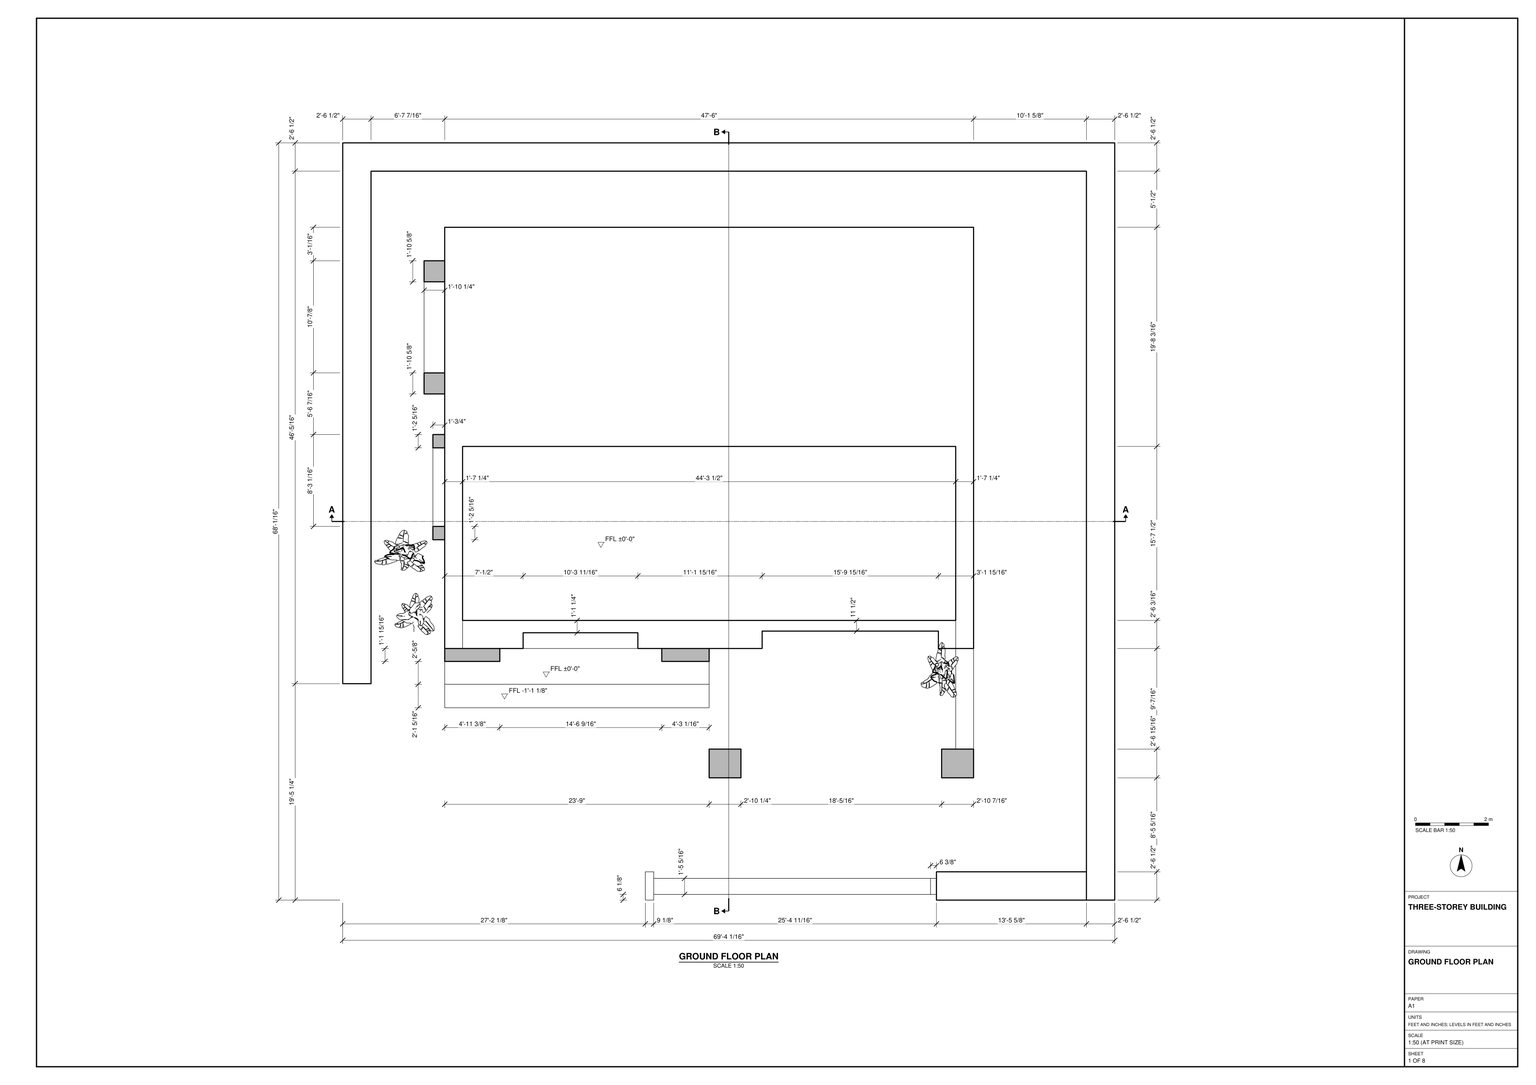
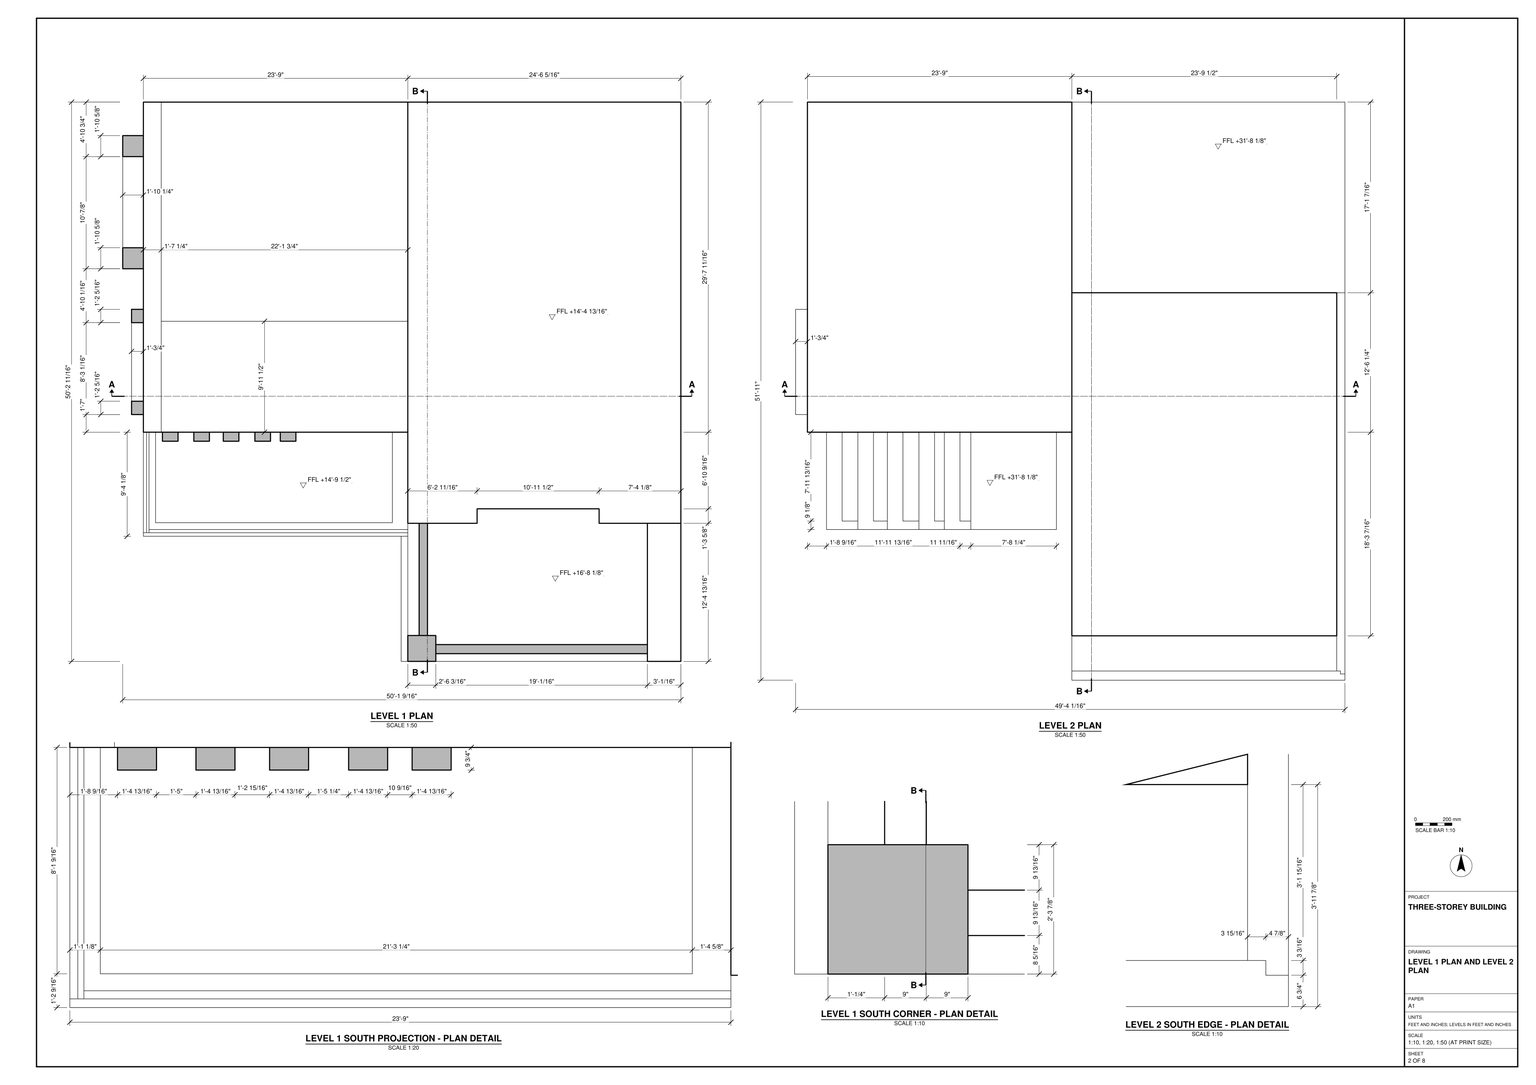
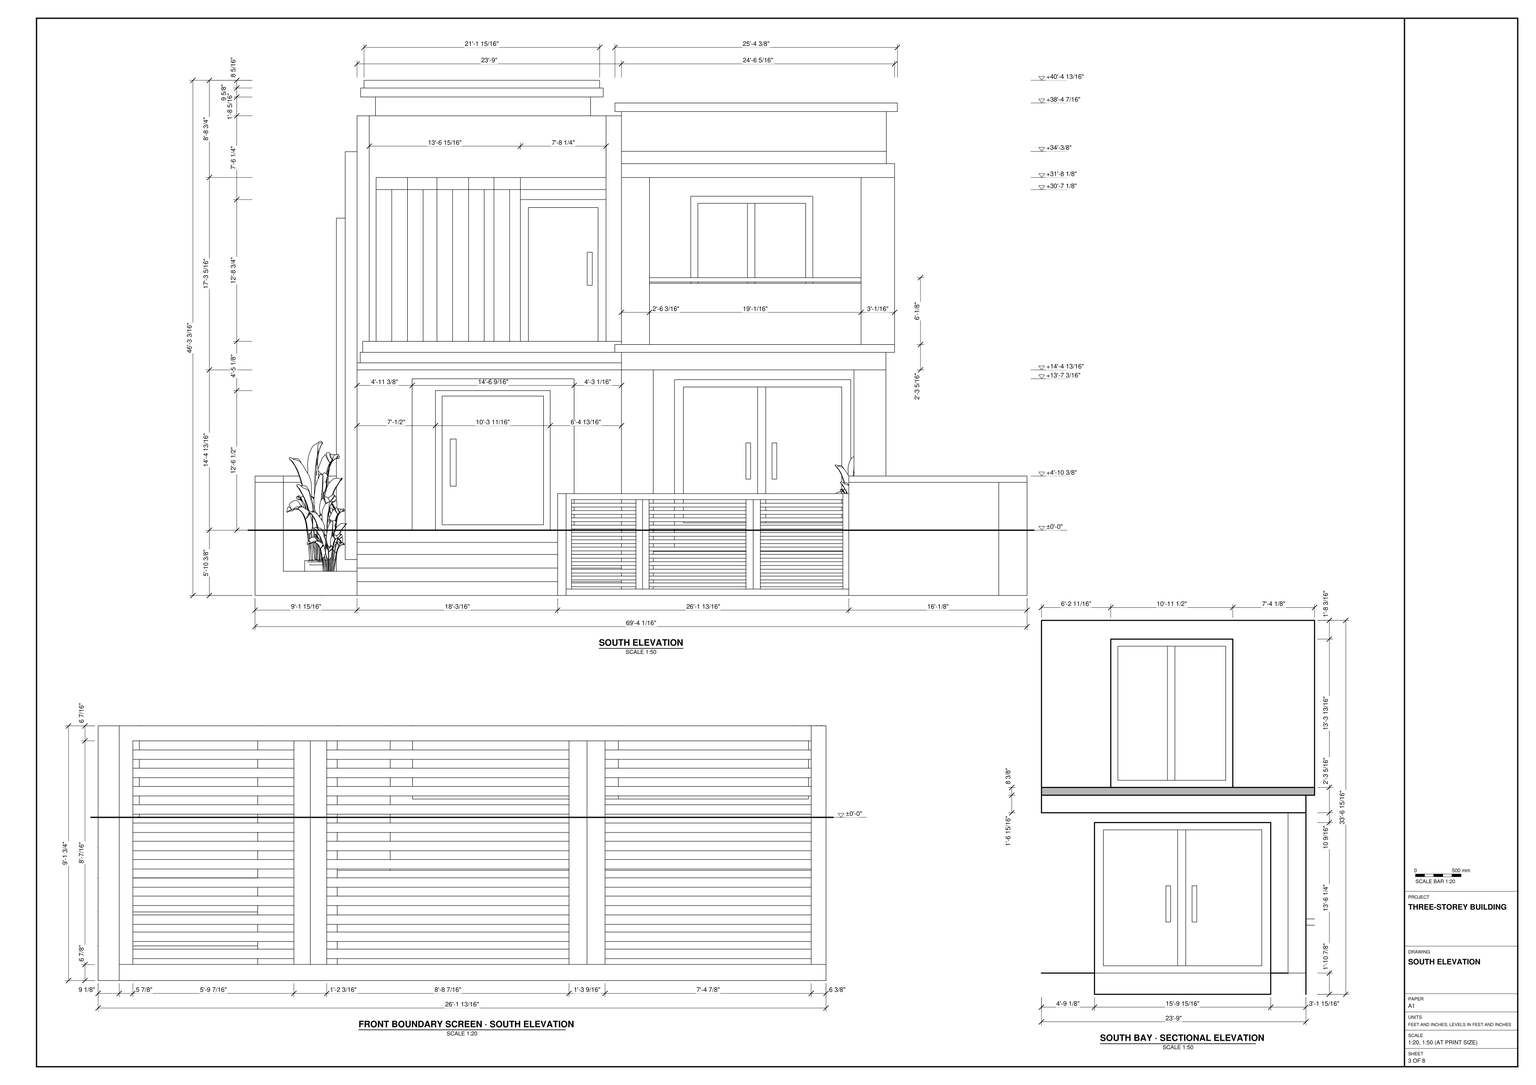
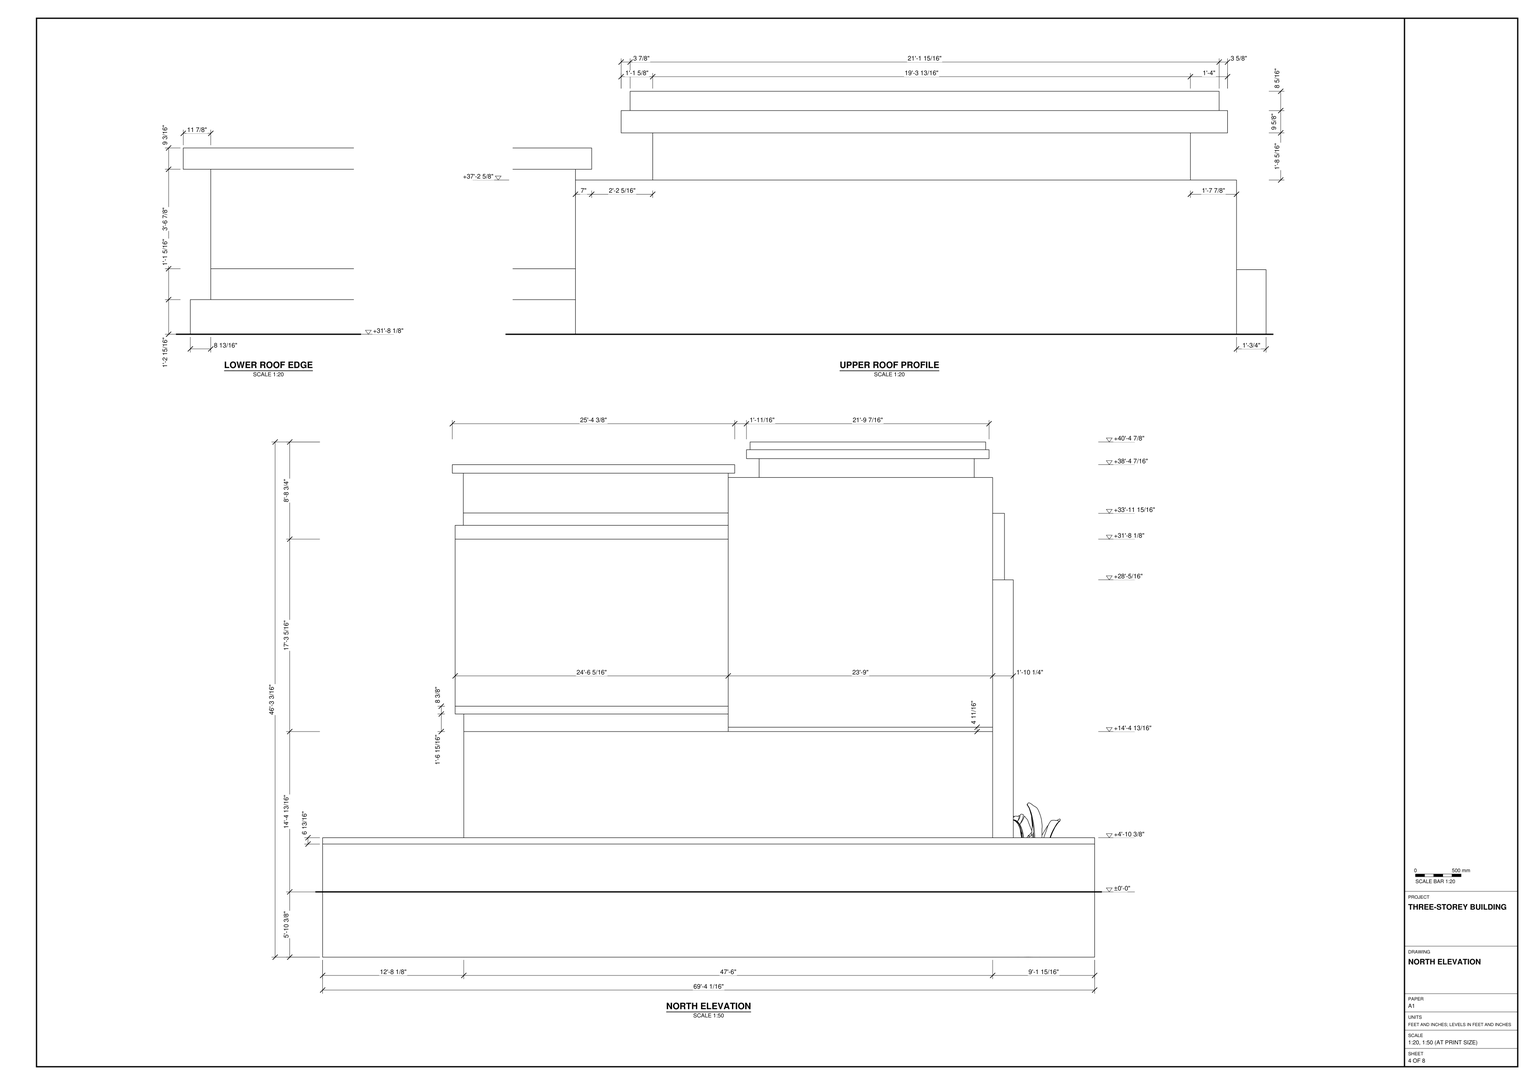
Build the three-storey building and its front court in SketchUp using task_files/diagram_01.pdf. Work in feet and inches. Include the site enclosure in the overall dimensions: 69'-4 1/16" along X, 68'-1/16" along Y and 46'-3 3/16" along Z. Set the ground floor at ±0'-0", Level 1 at +14'-4 13/16" and Level 2 at +31'-8 1/8".

Lay out the two adjoining bays from the plans. The east bay projects farther south, but the west bay has the higher roof cap. Model the walls at the thicknesses drawn, and use the sections and details to shape the floor slabs, projecting edges and roof caps. On the south face, distinguish the stepped approach to the single entrance from the paired doors in the adjoining bay. Above them, model the west projection with its vertical fins and the recessed east opening behind its low front wall. Follow the sheets for other openings, stairs and any built-in joinery or main furniture shown.

Extend the boundary walls around the site and place the slatted screen across the indicated part of the south frontage. Decor and loose items, including the plants beside the front court, may use any suitable library component. Keep shell elements such as walls, slabs and roof, and each furniture or joinery piece, in separate groups or components; use components for repeated parts. Save one SketchUp model as output_files/three_storey_building_with_a_slatted_boundary_screen.skp.

# SketchUp Ruby script. Lengths in inches.
U = 1.inch
M = Sketchup.active_model
def pt(a) = Geom::Point3d.new(a.map { |v| v * U })
def face(e, loops, mat)
  f = e.add_face(loops[0].map { |a| pt(a) })
  loops[1..].each { |l| e.add_face(l.map { |a| pt(a) }).erase! }
  f.material = f.back_material = mat if mat
  f
end
# faces: each face lists its corners as indices into pts; further lists are holes
def faces(e, pts, list, mat = nil) = list.each { |f| face(e, (f[0].is_a?(Array) ? f : [f]).map { |l| l.map { |i| pts[i] } }, mat) }
# xy, xz, yz: faces in a plane at the given z, y or x. An outline is a flat list of corners, or four numbers for a rectangle; further outlines are holes
def ring(l) = l.size == 4 ? [[l[0], l[1]], [l[2], l[1]], [l[2], l[3]], [l[0], l[3]]] : l.each_slice(2).to_a
def flat(e, list, mat, &to3) = list.each { |f| face(e, (f[0].is_a?(Array) ? f : [f]).map { |l| ring(l).map { |u, v| to3.(u, v) } }, mat) }
def xy(e, z, list, mat = nil) = flat(e, list, mat) { |x, y| [x, y, z] }
def xz(e, y, list, mat = nil) = flat(e, list, mat) { |x, z| [x, y, z] }
def yz(e, x, list, mat = nil) = flat(e, list, mat) { |y, z| [x, y, z] }
def lines(e, pts, list) = list.each { |a, b| e.add_line(pt(pts[a]), pt(pts[b])) }
# prism: a flat outline (further loops are holes) pulled along v
def prism(e, loops, v, mat = nil)
  f = face(e, loops, mat); d = Geom::Vector3d.new(v.map { |x| x * U })
  f.pushpull(f.normal.samedirection?(d) ? d.length : -d.length)
end
def box(e, o, s, mat = nil) = prism(e, [[o, [o[0] + s[0], o[1], o[2]], [o[0] + s[0], o[1] + s[1], o[2]], [o[0], o[1] + s[1], o[2]]]], [0, 0, s[2]], mat)
def at(x, y, z, deg = 0) = Geom::Transformation.translation(pt([x, y, z])) * Geom::Transformation.rotation(ORIGIN, Z_AXIS, deg.degrees)
def axes(o, x, y, z) = Geom::Transformation.new([*x, 0, *y, 0, *z, 0, *pt(o).to_a, 1])
def part(name) = M.definitions.add(name)
# library, detail: a bought-in or finely detailed component or shape, given as its bounding box
def library(name, o, s) = part(name).tap { |d| box(d.entities, o, s) }
def detail(e, o, s) = box(e.add_group.entities, o, s)
def put(e, d, t, mat = nil) = e.add_instance(d, t).tap { |i| i.material = mat if mat }
def group(e, t, mat = nil) = e.add_group.tap { |g| g.transformation = t; g.material = mat if mat }.entities
root = M.entities
M.materials.add("[0012_Bisque]").color = [255, 228, 196]
M.materials.add("[Asphalt New]").color = [94, 84, 87]
M.materials.add("[Asphalt New]1").color = [104, 93, 96]
M.materials.add("[Asphalt New]2").color = [117, 105, 108]
M.materials.add("[Carrera Marble]").color = [207, 207, 207]
M.materials.add("[Cladding Siding Tan]").color = [249, 194, 146]
M.materials.add("[Color M03]").color = [170, 170, 170]
M.materials.add("[Color M05]").color = [114, 114, 114]
M.materials.add("[Color M06]").color = [86, 86, 86]
M.materials.add("[Field Square Tile]").color = [217, 201, 169]
M.materials.add("[Formica Graystone]").color = [149, 146, 135]
M.materials.add("[Formica Laminate Dark]").color = [50, 53, 60]
M.materials.add("[Formica Laminate Light]").color = [213, 189, 164]
M.materials.add("[Formica Speckled Grey]").color = [94, 105, 111]
M.materials.add("[Leather Blue]").color = [45, 57, 74]
M.materials.add("[Marble Carrara Floor Tile]").color = [204, 208, 219]
M.materials.add("[Quartz Light Brown]").color = [199, 184, 152]
M.materials.add("[Terrazzo Tile Light]").color = [219, 217, 210]
M.materials.add("[Tile Travertine 2 inch]").color = [181, 178, 172]
M.materials.add("[Translucent Glass Gray]").color = [128, 128, 128]
M.materials["[Translucent Glass Gray]"].alpha = 0.5
M.materials.add("[Translucent Glass Safety]").color = [204, 235, 244]
M.materials["[Translucent Glass Safety]"].alpha = 0.23
M.materials.add("[Wood Bamboo]").color = [177, 105, 43]
M.materials.add("[Wood Cherry Original]").color = [152, 86, 42]
M.materials.add("[Wood Floor Light]").color = [204, 176, 127]
M.materials.add("[Wood Floor Parquet]").color = [145, 89, 39]
M.materials.add("[Wood Veneer 01]").color = [120, 70, 37]
c1 = library("chau cay",[-24.34,-109.24,0],[56.46,62.58,79.69])
xy(root,0,[[801.5625,0,801.5625,785.57,30.5,785.57,30.5,255,109.92,255,109.92,233.25,0,233.25,0,816.07,832.0625,816.07,832.0625,0],[326.12,0,335.21,30.5],[639.92,0,801.5625,30.5],[335.21,6.13,639.92,23.43],[335.21,23.43,639.92,30.5],
  [109.92,131.81,679.92,725.07],[87.67,545.5,109.92,689]])
xy(root,0,[[335.21,0,639.92,6.13]],"[Color M06]")
xy(root,0,[[0,0,0,233.25,30.5,233.25,30.5,30.5,326.12,30.5,326.12,0],[[30.5,30.5,30.5,233.25,109.92,233.25,109.92,255,30.5,255,30.5,785.57,801.5625,785.57,801.5625,30.5],[87.67,545.5,109.92,689]]],"[Tile Travertine 2 inch]")
xy(root,6.9375,[[335.21,6.13,341.09,23.43],[410.53,6.13,417.61,23.43],[417.61,6.13,424.69,23.43],[529.12,6.13,536.89,23.43],[536.89,6.13,544.66,23.43],
  [633.55,6.13,639.92,23.43]])
xy(root,6.9375,[[341.09,6.13,410.53,23.43],[424.69,6.13,529.12,23.43],[544.66,6.13,633.55,23.43]],"[Color M06]")
xy(root,9.46,[[341.09,11.38,633.55,18.2]])
xy(root,13.54,[[341.09,11.38,633.55,18.2]])
xy(root,14.95,[[109.92,150.43,394.92,271.17]])
xy(root,14.95,[[109.92,131.81,394.92,150.43]],"[Carrera Marble]")
xy(root,16.84,[[341.09,11.38,633.55,18.2]])
xy(root,20.92,[[341.09,11.38,633.55,18.2]])
xy(root,22.65,[[87.67,568.15,109.92,666.34]])
xy(root,24.21,[[341.09,11.38,633.55,18.2]])
xy(root,26.1,[[30.5,233.25,109.92,255]],"[Terrazzo Tile Light]")
xy(root,28.29,[[341.09,11.38,633.55,18.2]])
xy(root,29.58,[[109.92,180.46,394.92,271.17]])
xy(root,29.58,[[109.92,150.43,394.92,180.46]],"[Carrera Marble]")
xy(root,32.34,[[341.09,11.38,633.55,18.2]])
xy(root,36.42,[[341.09,11.38,633.55,18.2]])
xy(root,38.76,[[97.17,388.36,109.92,501.74]])
xy(root,40.21,[[341.09,11.38,633.55,18.2]])
xy(root,44.21,[[109.92,207.29,394.92,271.17]])
xy(root,44.21,[[109.92,180.46,394.92,207.29]],"[Carrera Marble]")
xy(root,44.29,[[341.09,11.38,633.55,18.2]])
xy(root,47.5,[[429.19,131.81,645.49,162.73],[394.92,162.73,660.68,162.73,660.68,271.17,641.98,271.17,641.98,289.9,452.05,289.9,452.05,271.17,394.92,271.17]],"[Field Square Tile]")
xy(root,48.09,[[341.09,11.38,633.55,18.2]])
xy(root,52.17,[[341.09,11.38,633.55,18.2]])
xy(root,53.09,[[97.17,402.7,109.92,487.41]])
xy(root,55.96,[[341.09,11.38,633.55,18.2]])
xy(root,57.22,[[109.92,232.61,394.92,271.17]])
xy(root,57.22,[[109.92,207.29,394.92,232.61]],"[Carrera Marble]")
xy(root,57.22,[[660.68,162.73,679.92,271.17]],"[Field Square Tile]")
xy(root,60.04,[[341.09,11.38,633.55,18.2]])
xy(root,63.84,[[341.09,11.38,633.55,18.2]])
xy(root,67.92,[[341.09,11.38,633.55,18.2]])
xy(root,70.36,[[109.92,257.23,129.17,271.17],[129.17,257.23,169.31,271.17],[343.875,257.23,394.92,271.17],[129.17,271.17,129.17,301.38,660.68,301.38,660.68,271.17,641.98,271.17,641.98,289.9,452.05,289.9,452.05,271.17,318.11,271.17,318.11,288.125,194.42,288.125,194.42,271.17],[129.17,301.38,660.68,488.89]])
xy(root,70.36,[[109.92,232.61,394.92,232.61,394.92,257.23,343.875,257.23,343.875,271.17,169.31,271.17,169.31,257.23,109.92,257.23],[194.42,271.17,318.11,288.125]],"[Carrera Marble]")
xy(root,71.51,[[87.67,568.15,109.92,666.34]],"[Asphalt New]2")
xy(root,71.71,[[341.09,11.38,633.55,18.2]])
xy(root,75.79,[[341.09,11.38,633.55,18.2]])
xy(root,79.59,[[341.09,11.38,633.55,18.2]])
xy(root,83.67,[[341.09,11.38,633.55,18.2]])
xy(root,84.1875,[[97.17,402.7,109.92,487.41]],"[Asphalt New]2")
xy(root,87.46,[[341.09,11.38,633.55,18.2]])
xy(root,91.54,[[341.09,11.38,633.55,18.2]])
xy(root,95.34,[[341.09,11.38,633.55,18.2]])
xy(root,99.42,[[341.09,11.38,633.55,18.2]])
xy(root,103.33,[[417.61,6.13,424.69,23.43],[536.89,6.13,544.66,23.43]])
xy(root,103.33,[[341.09,6.13,410.53,23.43],[424.69,6.13,529.12,23.43],[544.66,6.13,633.55,23.43]],"[Color M06]")
xy(root,109.8125,[[326.12,0,335.21,30.5],[335.21,6.13,633.55,23.43],[633.55,6.13,639.92,23.43]],"[Color M06]")
xy(root,121.9375,[[801.5625,0,801.5625,785.57,30.5,785.57,30.5,233.25,0,233.25,0,816.07,832.0625,816.07,832.0625,0],[639.92,0,801.5625,30.5]])
xy(root,128.75,[[639.92,0,832.0625,0,832.0625,816.07,0,816.07,0,233.25,30.5,233.25,30.5,785.57,801.5625,785.57,801.5625,30.5,639.92,30.5]],"[Formica Speckled Grey]")
xy(root,185.65,[[87.67,568.15,109.92,666.34]],"[Asphalt New]")
xy(root,197.53,[[97.17,402.7,109.92,487.41]],"[Asphalt New]")
xy(root,220.83,[[194.42,271.17,318.11,288.125]],"[Formica Speckled Grey]")
xy(root,232.61,[[452.05,271.17,641.98,289.9]])
xy(root,233.57,[[169.31,257.23,343.875,271.17]])
xy(root,243.14,[[394.92,131.81,429.19,162.73],[645.49,131.81,679.92,162.73],[109.92,257.23,394.92,271.17],[109.92,271.17,394.92,301.38],[394.92,271.17,679.92,301.38],
  [129.17,301.38,394.92,488.89],[394.92,301.38,660.68,488.89],[660.68,301.38,679.92,725.07],[129.17,488.89,394.92,725.07],[394.92,488.89,660.68,725.07]])
xy(root,243.14,[[429.19,131.81,429.19,162.73,394.92,162.73,394.92,271.17,679.92,271.17,679.92,162.73,645.49,162.73,645.49,131.81]],"[Asphalt New]")
xy(root,247.83,[[130.48,359.62,147.3,369.37],[164.29,359.62,181.11,369.37],[196.04,359.62,212.86,369.37],[230.11,359.62,246.93,369.37],[257.49,359.62,274.31,369.37]])
xy(root,247.83,[[123.06,271.8,378.29,271.8,378.29,369.37,274.31,369.37,274.31,359.62,257.49,359.62,257.49,369.37,246.93,369.37,246.93,359.62,230.11,359.62,230.11,369.37,212.86,369.37,212.86,359.62,196.04,359.62,196.04,369.37,181.11,369.37,181.11,359.62,164.29,359.62,164.29,369.37,147.3,369.37,147.3,359.62,130.48,359.62,130.48,369.37,123.06,369.37]],"[Leather Blue]")
xy(root,250.7,[[113.36,260.98,113.36,369.37,123.06,369.37,123.06,271.8,378.29,271.8,378.29,369.37,394.92,369.37,394.92,260.98]])
xy(root,250.7,[[109.92,257.23,394.92,260.98],[109.92,260.98,113.36,369.37]],"[Asphalt New]1")
xy(root,257.93,[[87.67,568.15,109.92,666.34]],"[Asphalt New]")
xy(root,262.05,[[394.92,131.81,679.92,725.07],[115.99,264.48,115.99,369.37,123.06,369.37,123.06,271.8,378.29,271.8,378.29,369.37,394.92,369.37,394.92,264.48],[679.92,271.17,689.23,725.07]])
xy(root,262.05,[[387.73,122.37,394.92,257.23],[394.92,122.37,689.23,131.81],[679.92,131.81,689.23,271.17]],"[Asphalt New]")
xy(root,262.05,[[113.36,260.98,115.99,369.37],[115.99,260.98,394.92,264.48]],"[Asphalt New]1")
xy(root,266.92,[[97.17,402.7,109.92,487.41]],"[Asphalt New]")
xy(root,270.46,[[394.92,122.37,425.11,150.25],[653.18,122.37,689.23,271.17],[425.11,130.68,653.18,140.46],[394.92,150.25,407.14,271.17],[407.14,150.25,416.125,271.17],
  [394.92,271.17,394.92,725.07,689.23,725.07,689.23,271.17,601.11,271.17,601.11,286.79,469.61,286.79,469.61,271.17]])
xy(root,270.46,[[387.73,122.37,394.92,257.23],[425.11,122.37,653.18,130.68]],"[Asphalt New]")
xy(root,270.46,[[425.11,140.46,653.18,140.46,653.18,271.17,601.11,271.17,601.11,286.79,469.61,286.79,469.61,271.17,416.125,271.17,416.125,150.25,425.11,150.25]],"[Marble Carrara Floor Tile]")
xy(root,273.93,[[115.99,264.48,394.92,264.48,394.92,369.37,378.29,369.37,378.29,271.8,123.06,271.8,123.06,369.37,115.99,369.37]],"[Asphalt New]1")
xy(root,336.46,[[425.11,130.68,653.18,140.46],[407.14,150.25,416.125,271.17]])
xy(root,356.91,[[87.67,568.15,109.92,666.34]])
xy(root,368.87,[[97.17,402.7,109.92,487.41]],"[Asphalt New]")
xy(root,406.64,[[87.67,545.5,109.92,689]])
xy(root,430.27,[[469.61,271.17,601.11,286.79]],"[Quartz Light Brown]")
xy(root,437.48,[[130.48,359.62,147.3,369.37],[164.29,359.62,181.11,369.37],[196.04,359.62,212.86,369.37],[230.11,359.62,246.93,369.37],[257.49,359.62,274.31,369.37]])
xy(root,437.48,[[130.48,264.48,130.48,359.62,147.3,359.62,147.3,273.58,164.29,273.58,164.29,264.48],[164.29,264.48,164.29,359.62,181.11,359.62,181.11,273.58,196.04,273.58,196.04,264.48],[196.04,264.48,196.04,359.62,212.86,359.62,212.86,273.58,230.11,273.58,230.11,264.48],[230.11,264.48,230.11,359.62,246.93,359.62,246.93,273.58,257.49,273.58,257.49,264.48],[257.49,264.48,257.49,359.62,274.31,359.62,274.31,273.58,286.01,273.58,286.01,264.48],
  [286.01,264.48,378.29,369.37]],"[Wood Bamboo]")
xy(root,450.46,[[394.92,122.37,425.11,150.25],[653.18,122.37,689.23,271.17],[394.92,271.17,689.23,519.64]])
xy(root,450.46,[[394.92,102.06,425.11,122.37],[425.11,102.06,425.11,150.25,394.92,150.25,394.92,271.17,653.18,271.17,653.18,102.06],[653.18,102.06,689.23,122.37]],"[Asphalt New]2")
xy(root,450.46,[[394.92,519.64,689.23,725.07]],"[Color M03]")
xy(root,450.46,[[130.48,264.48,164.29,264.48,164.29,273.58,147.3,273.58,147.3,369.37,130.48,369.37],[164.29,264.48,196.04,264.48,196.04,273.58,181.11,273.58,181.11,369.37,164.29,369.37],[196.04,264.48,230.11,264.48,230.11,273.58,212.86,273.58,212.86,369.37,196.04,369.37],[230.11,264.48,257.49,264.48,257.49,273.58,246.93,273.58,246.93,369.37,230.11,369.37],[257.49,264.48,286.01,264.48,286.01,273.58,274.31,273.58,274.31,369.37,257.49,369.37],
  [286.01,264.48,378.29,369.37]],"[Wood Bamboo]")
xy(root,463.99,[[97.17,402.7,109.92,487.41]])
xy(root,465.39,[[394.92,111.99,680.42,519.64]])
xy(root,465.39,[[394.92,102.06,394.92,111.99,684.36,111.99,684.36,108.81,689.23,108.81,689.23,102.06],[684.36,108.81,684.36,111.99,680.42,111.99,680.42,519.64,689.23,519.64,689.23,108.81]],"[Asphalt New]")
xy(root,478.32,[[97.17,388.36,109.92,501.74]])
xy(root,478.71,[[394.92,149.91,680.42,519.64]])
xy(root,478.71,[[394.92,111.99,680.42,149.91]],"[Asphalt New]")
xy(root,516.96,[[129.8,404.79,361.61,575.23]])
xy(root,516.96,[[[109.92,369.37,394.92,725.07],[129.8,404.79,361.61,575.23]]],"[Asphalt New]")
xy(root,521.58,[[394.92,149.91,680.42,519.64],[387.92,369.37,394.92,519.64]])
xy(root,521.58,[[387.92,137.41,394.92,369.37],[394.92,137.41,692.3,149.91],[680.42,149.91,692.3,519.64]],"[Asphalt New]")
xy(root,530.77,[[387.92,137.41,692.3,519.64]],"[Asphalt New]")
xy(root,537.27,[[129.8,404.79,361.61,575.23],[361.61,404.79,375.24,575.23]])
xy(root,537.27,[[113.8,375.54,129.8,594.36],[129.8,375.54,375.24,404.79],[129.8,575.23,375.24,594.36]],"[Asphalt New]")
xy(root,546.89,[[117.42,379.85,371.36,584.3]])
xy(root,546.89,[[[113.8,375.54,375.24,594.36],[117.42,379.85,371.36,584.3]]],"[Asphalt New]")
xy(root,555.21,[[117.42,379.85,371.36,584.3]],"[Asphalt New]")
xz(root,0,[[326.12,0,335.21,109.8125]],"[Color M06]")
xz(root,0,[[639.92,121.9375,832.0625,128.75]],"[Formica Speckled Grey]")
xz(root,0,[[639.92,0,801.5625,121.9375],[801.5625,0,832.0625,121.9375]],"[Terrazzo Tile Light]")
xz(root,6.13,[[335.21,0,639.92,6.9375],[335.21,6.9375,341.09,6.9375,341.09,103.33,633.55,103.33,633.55,109.8125,335.21,109.8125],[410.53,6.9375,417.61,103.33],[417.61,6.9375,424.69,103.33],[529.12,6.9375,536.89,103.33],
  [536.89,6.9375,544.66,103.33],[633.55,6.9375,639.92,109.8125]],"[Color M06]")
xz(root,11.38,[[341.09,9.46,633.55,13.54],[341.09,16.84,633.55,20.92],[341.09,24.21,633.55,28.29],[341.09,32.34,633.55,36.42],[341.09,40.21,633.55,44.29],
  [341.09,48.09,633.55,52.17],[341.09,55.96,633.55,60.04],[341.09,63.84,633.55,67.92],[341.09,71.71,633.55,75.79],[341.09,79.59,633.55,83.67],
  [341.09,87.46,633.55,91.54],[341.09,95.34,633.55,99.42]],"[Color M05]")
xz(root,18.2,[[341.09,9.46,633.55,13.54],[341.09,16.84,633.55,20.92],[341.09,24.21,633.55,28.29],[341.09,32.34,633.55,36.42],[341.09,40.21,633.55,44.29],
  [341.09,48.09,633.55,52.17],[341.09,55.96,633.55,60.04],[341.09,63.84,633.55,67.92],[341.09,71.71,633.55,75.79],[341.09,79.59,633.55,83.67],
  [341.09,87.46,633.55,91.54],[341.09,95.34,633.55,99.42]],"[Color M05]")
xz(root,23.43,[[335.21,0,639.92,6.9375],[335.21,6.9375,335.21,109.8125,633.55,109.8125,633.55,103.33,341.09,103.33,341.09,6.9375],[410.53,6.9375,417.61,103.33],[417.61,6.9375,424.69,103.33],[529.12,6.9375,536.89,103.33],
  [536.89,6.9375,544.66,103.33],[633.55,6.9375,639.92,109.8125]],"[Color M06]")
xz(root,30.5,[[326.12,0,335.21,109.8125]],"[Color M06]")
xz(root,30.5,[[639.92,121.9375,801.5625,128.75]],"[Formica Speckled Grey]")
xz(root,30.5,[[639.92,0,801.5625,121.9375]],"[Terrazzo Tile Light]")
xz(root,102.06,[[394.92,450.46,689.23,465.39]],"[Asphalt New]")
xz(root,111.99,[[394.92,465.39,680.42,478.71]],"[Asphalt New]")
xz(root,122.37,[[394.92,270.46,425.11,450.46],[653.18,270.46,689.23,450.46]])
xz(root,122.37,[[387.73,262.05,689.23,270.46]],"[Asphalt New]")
xz(root,130.68,[[425.11,270.46,653.18,336.46]],"[Translucent Glass Safety]")
xz(root,131.81,[[394.92,0,429.19,243.14],[645.49,0,679.92,243.14]])
xz(root,131.81,[[394.92,243.14,679.92,262.05]],"[Asphalt New]")
xz(root,131.81,[[109.92,0,394.92,14.95]],"[Carrera Marble]")
xz(root,131.81,[[429.19,0,645.49,47.5]],"[Field Square Tile]")
xz(root,137.41,[[387.92,521.58,692.3,530.77]],"[Asphalt New]")
xz(root,140.46,[[425.11,270.46,653.18,336.46]],"[Translucent Glass Safety]")
xz(root,149.91,[[394.92,478.71,680.42,521.58]],"[Asphalt New]")
xz(root,150.25,[[[394.92,270.46,394.92,450.46,425.11,450.46,425.11,270.46,416.125,270.46,416.125,336.46,407.14,336.46,407.14,270.46],[410.6,337.75,411.05,337.81,411.47,337.98,411.83,338.26,412.11,338.62,412.29,339.04,412.35,339.5,412.29,339.95,412.11,340.37,411.83,340.74,411.47,341.01,411.05,341.1875,410.6,341.25,410.14,341.1875,409.72,341.01,409.36,340.74,409.08,340.37,408.91,339.95,408.85,339.5,408.91,339.04,409.08,338.62,409.36,338.26,409.72,337.98,410.14,337.81]],[407.14,270.46,416.125,336.46],[410.6,337.75,411.05,337.81,411.47,337.98,411.83,338.26,412.11,338.62,412.29,339.04,412.35,339.5,412.29,339.95,412.11,340.37,411.83,340.74,411.47,341.01,411.05,341.1875,410.6,341.25,410.14,341.1875,409.72,341.01,409.36,340.74,409.08,340.37,408.91,339.95,408.85,339.5,408.91,339.04,409.08,338.62,409.36,338.26,409.72,337.98,410.14,337.81]])
xz(root,150.43,[[109.92,14.95,394.92,29.58]],"[Carrera Marble]")
xz(root,162.73,[[394.92,47.5,429.19,243.14],[645.49,47.5,645.49,243.14,679.92,243.14,679.92,57.22,660.68,57.22,660.68,47.5]])
xz(root,180.46,[[109.92,29.58,394.92,44.21]],"[Carrera Marble]")
xz(root,207.29,[[109.92,44.21,394.92,57.22]],"[Carrera Marble]")
xz(root,232.61,[[109.92,57.22,394.92,70.36]],"[Carrera Marble]")
xz(root,233.25,[[0,121.9375,30.5,128.75]],"[Formica Speckled Grey]")
xz(root,233.25,[[0,0,109.92,0,109.92,26.1,30.5,26.1,30.5,121.9375,0,121.9375]],"[Terrazzo Tile Light]")
xz(root,255,[[30.5,0,109.92,26.1]])
xz(root,257.23,[[109.92,70.36,169.31,70.36,169.31,233.57,343.875,233.57,343.875,70.36,394.92,70.36,394.92,243.14,109.92,243.14],[387.73,262.05,394.92,270.46]])
xz(root,257.23,[[109.92,243.14,394.92,250.7]],"[Asphalt New]1")
xz(root,260.98,[[113.36,250.7,394.92,262.05]],"[Asphalt New]1")
xz(root,264.48,[[115.99,262.05,394.92,273.93]],"[Asphalt New]1")
xz(root,264.48,[[130.48,437.48,164.29,450.46],[164.29,437.48,196.04,450.46],[196.04,437.48,230.11,450.46],[230.11,437.48,257.49,450.46],[257.49,437.48,286.01,450.46],
  [286.01,437.48,378.29,450.46]],"[Wood Bamboo]")
xz(root,271.17,[[109.92,14.95,394.92,29.58],[109.92,29.58,394.92,44.21],[109.92,44.21,394.92,57.22],[109.92,57.22,394.92,70.36],[109.92,70.36,109.92,243.14,394.92,243.14,394.92,70.36,343.875,70.36,343.875,233.57,169.31,233.57,169.31,70.36],
  [407.14,270.46,416.125,336.46],[653.18,270.46,689.23,450.46]])
xz(root,271.17,[[394.92,47.5,452.05,70.36],[641.98,47.5,660.68,70.36],[660.68,57.22,679.92,70.36],[169.31,70.36,194.42,70.36,194.42,220.83,318.11,220.83,318.11,70.36,343.875,70.36,343.875,233.57,169.31,233.57],[394.92,70.36,452.05,70.36,452.05,232.61,641.98,232.61,641.98,70.36,679.92,70.36,679.92,243.14,394.92,243.14],
  [[394.92,270.46,407.14,270.46,407.14,336.46,416.125,336.46,416.125,270.46,469.61,270.46,469.61,430.27,601.11,430.27,601.11,270.46,653.18,270.46,653.18,450.46,394.92,450.46],[410.6,337.75,410.14,337.81,409.72,337.98,409.36,338.26,409.08,338.62,408.91,339.04,408.85,339.5,408.91,339.95,409.08,340.37,409.36,340.74,409.72,341.01,410.14,341.1875,410.6,341.25,411.05,341.1875,411.47,341.01,411.83,340.74,412.11,340.37,412.29,339.95,412.35,339.5,412.29,339.04,412.11,338.62,411.83,338.26,411.47,337.98,411.05,337.81]]],"[Formica Speckled Grey]")
xz(root,271.8,[[123.06,247.83,378.29,250.7],[123.06,250.7,378.29,262.05],[123.06,262.05,378.29,273.93]],"[Asphalt New]1")
xz(root,273.58,[[147.3,437.48,164.29,450.46],[181.11,437.48,196.04,450.46],[212.86,437.48,230.11,450.46],[246.93,437.48,257.49,450.46],[274.31,437.48,286.01,450.46]])
xz(root,286.79,[[477.25,278.09,530.71,422.63],[538.69,278.09,593.48,422.63]],"[Formica Laminate Light]")
xz(root,286.79,[[[469.61,270.46,601.11,430.27],[477.25,278.09,593.48,422.63]],[530.71,278.09,538.69,422.63]],"[Wood Veneer 01]")
xz(root,288.125,[[[201.59,76.23,310.94,214.95],[210.35,117.78,216.79,168.68]]],"[Cladding Siding Tan]")
xz(root,288.125,[[210.35,117.78,216.79,168.68]],"[Formica Graystone]")
xz(root,288.125,[[[194.42,70.36,318.11,220.83],[201.59,76.23,310.94,214.95]]],"[Formica Laminate Light]")
xz(root,289.9,[[529.04,125.43,534.1,164.4375],[557.22,125.43,562.29,164.4375]],"[Formica Graystone]")
xz(root,289.9,[[452.05,47.5,641.98,70.36]],"[Formica Speckled Grey]")
xz(root,289.9,[[[461.67,78.25,541.6,224.72],[529.04,125.43,534.1,164.4375]],[[550.4,78.25,632.36,224.72],[557.22,125.43,562.29,164.4375]]],"[Wood Floor Light]")
xz(root,289.9,[[[452.05,70.36,641.98,232.61],[461.67,78.25,632.36,224.72]],[541.6,78.25,550.4,224.72]],"[Wood Veneer 01]")
xz(root,301.38,[[129.17,70.36,660.68,243.14]])
xz(root,359.62,[[130.48,247.83,147.3,437.48],[164.29,247.83,181.11,437.48],[196.04,247.83,212.86,437.48],[230.11,247.83,246.93,437.48],[257.49,247.83,274.31,437.48]],"[Wood Bamboo]")
xz(root,369.37,[[109.92,247.83,123.06,250.7],[130.48,247.83,147.3,437.48],[164.29,247.83,181.11,437.48],[196.04,247.83,212.86,437.48],[230.11,247.83,246.93,437.48],
  [257.49,247.83,274.31,437.48],[378.29,247.83,394.92,250.7],[113.36,250.7,123.06,262.05],[378.29,250.7,394.92,262.05],[115.99,262.05,123.06,273.93],
  [378.29,262.05,394.92,273.93],[130.48,437.48,147.3,450.46],[164.29,437.48,181.11,450.46],[196.04,437.48,212.86,450.46],[230.11,437.48,246.93,450.46],
  [257.49,437.48,274.31,450.46],[286.01,437.48,378.29,450.46]])
xz(root,369.37,[[147.3,247.83,164.29,450.46],[181.11,247.83,196.04,450.46],[212.86,247.83,230.11,450.46],[246.93,247.83,257.49,450.46],[274.31,247.83,286.01,450.46],
  [286.01,426.69,378.29,437.48]],"[0012_Bisque]")
xz(root,369.37,[[123.06,247.83,130.48,247.83,130.48,450.46,378.29,450.46,378.29,516.96,123.06,516.96],[109.92,250.7,113.36,250.7,113.36,262.05,115.99,262.05,115.99,273.93,123.06,273.93,123.06,516.96,109.92,516.96],[378.29,273.93,394.92,516.96]],"[Asphalt New]")
xz(root,369.37,[[357.95,334.27,363.45,369.9]],"[Formica Speckled Grey]")
xz(root,369.37,[[[286.01,247.83,378.29,426.69],[294.61,256.43,369.6875,418.09]],[[294.61,256.43,369.6875,418.09],[357.95,334.27,363.45,369.9]]],"[Wood Floor Parquet]")
xz(root,375.54,[[113.8,537.27,375.24,546.89]],"[Asphalt New]")
xz(root,379.85,[[117.42,546.89,371.36,555.21]],"[Asphalt New]")
xz(root,388.36,[[97.17,38.76,109.92,478.32]])
xz(root,402.7,[[97.17,53.09,109.92,84.1875],[97.17,197.53,109.92,266.92],[97.17,368.87,109.92,463.99]])
xz(root,402.7,[[97.17,84.1875,109.92,197.53],[97.17,266.92,109.92,368.87]],"[Formica Graystone]")
xz(root,404.79,[[129.8,516.96,361.61,537.27]],"[Asphalt New]")
xz(root,487.41,[[97.17,53.09,109.92,84.1875],[97.17,197.53,109.92,266.92],[97.17,368.87,109.92,463.99]])
xz(root,487.41,[[97.17,84.1875,109.92,197.53],[97.17,266.92,109.92,368.87]],"[Formica Graystone]")
xz(root,488.89,[[129.17,70.36,660.68,243.14]])
xz(root,501.74,[[97.17,38.76,109.92,478.32]])
xz(root,519.64,[[394.92,450.46,689.23,465.39],[394.92,465.39,680.42,478.71],[394.92,478.71,680.42,521.58],[387.92,521.58,692.3,530.77]],"[Asphalt New]")
xz(root,545.5,[[87.67,0,109.92,406.64]])
xz(root,568.15,[[87.67,22.65,109.92,71.51],[87.67,185.65,109.92,257.93]])
xz(root,568.15,[[87.67,71.51,109.92,185.65],[87.67,257.93,109.92,356.91]],"[Formica Graystone]")
xz(root,575.23,[[129.8,516.96,361.61,537.27]],"[Asphalt New]")
xz(root,584.3,[[117.42,546.89,371.36,555.21]],"[Asphalt New]")
xz(root,594.36,[[113.8,537.27,375.24,546.89]],"[Asphalt New]")
xz(root,666.34,[[87.67,22.65,109.92,71.51],[87.67,185.65,109.92,257.93]])
xz(root,666.34,[[87.67,71.51,109.92,185.65],[87.67,257.93,109.92,356.91]],"[Formica Graystone]")
xz(root,689,[[87.67,0,109.92,406.64]])
xz(root,725.07,[[109.92,247.83,394.92,516.96]],"[Asphalt New]2")
xz(root,725.07,[[109.92,0,679.92,70.36],[109.92,70.36,679.92,243.14],[109.92,243.14,394.92,247.83],[394.92,243.14,679.92,262.05],[394.92,262.05,689.23,270.46],
  [394.92,270.46,689.23,450.46]],"[Color M03]")
xz(root,785.57,[[30.5,121.9375,801.5625,128.75]],"[Formica Speckled Grey]")
xz(root,785.57,[[30.5,0,801.5625,121.9375]],"[Terrazzo Tile Light]")
xz(root,816.07,[[0,121.9375,832.0625,128.75]],"[Formica Speckled Grey]")
xz(root,816.07,[[0,0,832.0625,121.9375]],"[Terrazzo Tile Light]")
yz(root,0,[[233.25,121.9375,816.07,128.75]],"[Formica Speckled Grey]")
yz(root,0,[[233.25,0,816.07,121.9375]],"[Terrazzo Tile Light]")
yz(root,30.5,[[233.25,121.9375,255,128.75],[255,121.9375,785.57,128.75]],"[Formica Speckled Grey]")
yz(root,30.5,[[255,0,785.57,121.9375],[233.25,26.1,255,121.9375]],"[Terrazzo Tile Light]")
yz(root,87.67,[[[545.5,0,689,406.64],[568.15,22.65,666.34,356.91]]])
yz(root,87.67,[[568.15,185.65,666.34,257.93]],"[Asphalt New]")
yz(root,87.67,[[568.15,22.65,666.34,71.51]],"[Asphalt New]2")
yz(root,97.17,[[[388.36,38.76,501.74,478.32],[402.7,53.09,487.41,463.99]]])
yz(root,97.17,[[402.7,197.53,487.41,266.92],[402.7,368.87,487.41,463.99]],"[Asphalt New]")
yz(root,97.17,[[402.7,53.09,487.41,84.1875]],"[Asphalt New]2")
yz(root,109.92,[[233.25,0,255,14.95],[[545.5,0,689,406.64],[568.15,22.65,666.34,356.91]],[233.25,14.95,255,26.1],[568.15,22.65,666.34,71.51],[[388.36,38.76,501.74,478.32],[402.7,53.09,487.41,463.99]],
  [402.7,53.09,487.41,84.1875],[257.23,70.36,271.17,243.14],[568.15,185.65,666.34,257.93],[402.7,197.53,487.41,266.92],[402.7,368.87,487.41,463.99]])
yz(root,109.92,[[[255,0,255,14.95,271.17,14.95,271.17,243.14,369.37,243.14,369.37,516.96,725.07,516.96,725.07,0,689,0,689,406.64,545.5,406.64,545.5,0],[388.36,38.76,501.74,478.32]]],"[Asphalt New]")
yz(root,109.92,[[257.23,243.14,369.37,250.7]],"[Asphalt New]1")
yz(root,109.92,[[131.81,0,233.25,14.95],[150.43,14.95,150.43,29.58,271.17,29.58,271.17,14.95,255,14.95,255,26.1,233.25,26.1,233.25,14.95],[180.46,29.58,271.17,44.21],[207.29,44.21,271.17,57.22],[232.61,57.22,271.17,70.36]],"[Carrera Marble]")
yz(root,109.92,[[402.7,365.45,487.41,368.87]],"[Formica Graystone]")
yz(root,109.92,[[[568.15,71.51,666.34,185.65],[576.52,79.875,657.98,177.28]],[615.52,79.875,623,177.28],[[402.7,84.1875,487.41,197.53],[411.05,92.54,479.05,189.18]],[442.9375,92.54,450.125,189.18],[[568.15,257.93,666.34,356.91],[575.06,264.84,659.43,350]],
  [617.48,264.84,623.92,350],[[402.7,266.92,487.41,365.45],[410.2,274.42,479.9,357.94]],[442.9375,274.42,450.125,357.94]],"[Formica Laminate Dark]")
yz(root,109.92,[[576.52,79.875,615.52,177.28],[623,79.875,657.98,177.28],[411.05,92.54,442.9375,189.18],[450.125,92.54,479.05,189.18],[575.06,264.84,617.48,350],
  [623.92,264.84,659.43,350],[410.2,274.42,442.9375,357.94],[450.125,274.42,479.9,357.94]],"[Translucent Glass Gray]")
yz(root,113.36,[[260.98,250.7,369.37,262.05]],"[Asphalt New]1")
yz(root,113.8,[[375.54,537.27,594.36,546.89]],"[Asphalt New]")
yz(root,115.99,[[264.48,262.05,369.37,273.93]],"[Asphalt New]1")
yz(root,117.42,[[379.85,546.89,584.3,555.21]],"[Asphalt New]")
yz(root,123.06,[[271.8,247.83,369.37,250.7],[271.8,250.7,369.37,262.05],[271.8,262.05,369.37,273.93]],"[Asphalt New]1")
yz(root,129.17,[[301.38,70.36,488.89,243.14]])
yz(root,129.8,[[404.79,516.96,575.23,537.27]],"[Asphalt New]")
yz(root,130.48,[[359.62,247.83,369.37,437.48],[264.48,437.48,369.37,450.46]],"[Wood Bamboo]")
yz(root,147.3,[[359.62,247.83,369.37,437.48],[273.58,437.48,369.37,450.46]],"[Wood Bamboo]")
yz(root,164.29,[[359.62,247.83,369.37,437.48],[273.58,437.48,369.37,450.46]],"[Wood Bamboo]")
yz(root,169.31,[[257.23,70.36,271.17,233.57]])
yz(root,181.11,[[359.62,247.83,369.37,437.48],[273.58,437.48,369.37,450.46]],"[Wood Bamboo]")
yz(root,194.42,[[271.17,70.36,288.125,220.83]],"[Formica Speckled Grey]")
yz(root,196.04,[[359.62,247.83,369.37,437.48],[273.58,437.48,369.37,450.46]],"[Wood Bamboo]")
yz(root,212.86,[[359.62,247.83,369.37,437.48],[273.58,437.48,369.37,450.46]],"[Wood Bamboo]")
yz(root,230.11,[[359.62,247.83,369.37,437.48],[273.58,437.48,369.37,450.46]],"[Wood Bamboo]")
yz(root,246.93,[[359.62,247.83,369.37,437.48],[273.58,437.48,369.37,450.46]],"[Wood Bamboo]")
yz(root,257.49,[[359.62,247.83,369.37,437.48],[273.58,437.48,369.37,450.46]],"[Wood Bamboo]")
yz(root,274.31,[[359.62,247.83,369.37,437.48],[273.58,437.48,369.37,450.46]],"[Wood Bamboo]")
yz(root,286.01,[[273.58,437.48,369.37,450.46]],"[Wood Bamboo]")
yz(root,318.11,[[271.17,70.36,288.125,220.83]],"[Formica Speckled Grey]")
yz(root,326.12,[[0,0,30.5,109.8125]],"[Color M06]")
yz(root,335.21,[[6.13,0,23.43,6.9375],[6.13,6.9375,23.43,109.8125]])
yz(root,335.21,[[0,0,6.13,109.8125],[23.43,0,30.5,109.8125]],"[Color M06]")
yz(root,341.09,[[11.38,9.46,18.2,13.54],[11.38,16.84,18.2,20.92],[11.38,24.21,18.2,28.29],[11.38,32.34,18.2,36.42],[11.38,40.21,18.2,44.29],
  [11.38,48.09,18.2,52.17],[11.38,55.96,18.2,60.04],[11.38,63.84,18.2,67.92],[11.38,71.71,18.2,75.79],[11.38,79.59,18.2,83.67],
  [11.38,87.46,18.2,91.54],[11.38,95.34,18.2,99.42]])
yz(root,341.09,[[[6.13,6.9375,23.43,103.33],[11.38,95.34,18.2,99.42],[11.38,87.46,18.2,91.54],[11.38,79.59,18.2,83.67],[11.38,71.71,18.2,75.79],[11.38,63.84,18.2,67.92],[11.38,55.96,18.2,60.04],[11.38,48.09,18.2,52.17],[11.38,40.21,18.2,44.29],[11.38,32.34,18.2,36.42],[11.38,9.46,18.2,13.54],[11.38,24.21,18.2,28.29],[11.38,16.84,18.2,20.92]]],"[Color M06]")
yz(root,343.875,[[257.23,70.36,271.17,233.57]])
yz(root,361.61,[[404.79,516.96,575.23,537.27]],"[Asphalt New]")
yz(root,371.36,[[379.85,546.89,584.3,555.21]],"[Asphalt New]")
yz(root,375.24,[[375.54,537.27,594.36,546.89]],"[Asphalt New]")
yz(root,378.29,[[271.8,247.83,369.37,250.7],[271.8,250.7,369.37,262.05],[271.8,262.05,369.37,273.93]],"[Asphalt New]1")
yz(root,378.29,[[264.48,437.48,369.37,450.46]],"[Wood Cherry Original]")
yz(root,387.73,[[122.37,262.05,257.23,270.46]],"[Asphalt New]")
yz(root,387.92,[[137.41,521.58,519.64,530.77]],"[Asphalt New]")
yz(root,394.92,[[131.81,14.95,131.81,243.14,162.73,243.14,162.73,29.58,150.43,29.58,150.43,14.95],[150.43,14.95,162.73,29.58],[162.73,14.95,271.17,29.58],[180.46,29.58,271.17,44.21],[207.29,44.21,271.17,47.5],
  [257.23,70.36,271.17,243.14],[257.23,243.14,257.23,250.7,369.37,250.7,369.37,247.83,725.07,247.83,725.07,243.14],[369.37,247.83,725.07,262.05],[260.98,250.7,369.37,262.05],[257.23,258.33,260.98,262.05],
  [257.23,262.05,264.48,270.46],[264.48,262.05,369.37,270.46],[369.37,262.05,725.07,270.46],[122.37,270.46,150.25,450.46],[264.48,270.46,271.17,273.93],
  [271.17,270.46,369.37,273.93],[369.37,270.46,725.07,450.46],[369.37,450.46,519.64,465.39],[369.37,465.39,519.64,478.71],[369.37,478.71,519.64,516.96],
  [369.37,516.96,519.64,521.58]])
yz(root,394.92,[[131.81,243.14,131.81,262.05,257.23,262.05,257.23,258.33,260.98,258.33,260.98,250.7,257.23,250.7,257.23,243.14],[102.06,450.46,369.37,465.39],[111.99,465.39,369.37,478.71],[149.91,478.71,369.37,521.58]],"[Asphalt New]")
yz(root,394.92,[[519.64,450.46,725.07,516.96]],"[Asphalt New]2")
yz(root,394.92,[[207.29,47.5,232.61,57.22],[232.61,47.5,271.17,57.22],[232.61,57.22,271.17,70.36]],"[Carrera Marble]")
yz(root,394.92,[[162.73,29.58,162.73,47.5,207.29,47.5,207.29,44.21,180.46,44.21,180.46,29.58]],"[Field Square Tile]")
yz(root,394.92,[[271.17,273.93,369.37,450.46]],"[Formica Speckled Grey]")
yz(root,407.14,[[150.25,270.46,271.17,336.46]],"[Translucent Glass Safety]")
yz(root,410.53,[[6.13,6.9375,23.43,103.33]],"[Color M06]")
yz(root,416.125,[[150.25,270.46,271.17,336.46]],"[Translucent Glass Safety]")
yz(root,417.61,[[6.13,6.9375,23.43,103.33]])
yz(root,424.69,[[6.13,6.9375,23.43,103.33]],"[Color M06]")
yz(root,425.11,[[[122.37,270.46,130.68,270.46,130.68,336.46,140.46,336.46,140.46,270.46,150.25,270.46,150.25,450.46,122.37,450.46],[135.14,337.83,134.53,337.91,133.96,338.14,133.46,338.52,133.09,339.01,132.85,339.59,132.77,340.2,132.85,340.82,133.09,341.39,133.46,341.88,133.96,342.26,134.53,342.5,135.14,342.58,135.76,342.5,136.33,342.26,136.82,341.88,137.2,341.39,137.4375,340.82,137.52,340.2,137.4375,339.59,137.2,339.01,136.82,338.52,136.33,338.14,135.76,337.91]],[130.68,270.46,140.46,336.46],[135.14,337.83,134.53,337.91,133.96,338.14,133.46,338.52,133.09,339.01,132.85,339.59,132.77,340.2,132.85,340.82,133.09,341.39,133.46,341.88,133.96,342.26,134.53,342.5,135.14,342.58,135.76,342.5,136.33,342.26,136.82,341.88,137.2,341.39,137.4375,340.82,137.52,340.2,137.4375,339.59,137.2,339.01,136.82,338.52,136.33,338.14,135.76,337.91]])
yz(root,429.19,[[131.81,47.5,162.73,243.14]])
yz(root,452.05,[[271.17,47.5,289.9,70.36],[271.17,70.36,289.9,232.61]],"[Formica Speckled Grey]")
yz(root,469.61,[[271.17,270.46,286.79,430.27]],"[Quartz Light Brown]")
yz(root,529.12,[[6.13,6.9375,23.43,103.33]],"[Color M06]")
yz(root,536.89,[[6.13,6.9375,23.43,103.33]])
yz(root,544.66,[[6.13,6.9375,23.43,103.33]],"[Color M06]")
yz(root,601.11,[[271.17,270.46,286.79,430.27]],"[Quartz Light Brown]")
yz(root,633.55,[[[6.13,6.9375,23.43,103.33],[11.38,95.34,18.2,99.42],[11.38,87.46,18.2,91.54],[11.38,79.59,18.2,83.67],[11.38,71.71,18.2,75.79],[11.38,63.84,18.2,67.92],[11.38,55.96,18.2,60.04],[11.38,48.09,18.2,52.17],[11.38,40.21,18.2,44.29],[11.38,32.34,18.2,36.42],[11.38,24.21,18.2,28.29],[11.38,16.84,18.2,20.92],[11.38,9.46,18.2,13.54]]],"[Color M06]")
yz(root,639.92,[[6.13,0,23.43,6.9375],[6.13,6.9375,23.43,109.8125]])
yz(root,639.92,[[0,121.9375,30.5,128.75]],"[Formica Speckled Grey]")
yz(root,639.92,[[0,0,0,121.9375,30.5,121.9375,30.5,0,23.43,0,23.43,109.8125,6.13,109.8125,6.13,0]],"[Terrazzo Tile Light]")
yz(root,641.98,[[271.17,47.5,289.9,70.36],[271.17,70.36,289.9,232.61]],"[Formica Speckled Grey]")
yz(root,645.49,[[131.81,47.5,162.73,243.14]])
yz(root,653.18,[[[122.37,270.46,122.37,450.46,271.17,450.46,271.17,270.46,140.46,270.46,140.46,336.46,130.68,336.46,130.68,270.46],[135.14,337.83,135.76,337.91,136.33,338.14,136.82,338.52,137.2,339.01,137.4375,339.59,137.52,340.2,137.4375,340.82,137.2,341.39,136.82,341.88,136.33,342.26,135.76,342.5,135.14,342.58,134.53,342.5,133.96,342.26,133.46,341.88,133.09,341.39,132.85,340.82,132.77,340.2,132.85,339.59,133.09,339.01,133.46,338.52,133.96,338.14,134.53,337.91]],[130.68,270.46,140.46,336.46]])
yz(root,660.68,[[301.38,70.36,488.89,243.14]])
yz(root,660.68,[[162.73,47.5,271.17,57.22]],"[Field Square Tile]")
yz(root,679.92,[[131.81,0,162.73,243.14]])
yz(root,679.92,[[131.81,243.14,271.17,262.05]],"[Asphalt New]")
yz(root,679.92,[[271.17,0,725.07,70.36],[271.17,70.36,725.07,243.14],[271.17,243.14,725.07,262.05]],"[Color M03]")
yz(root,679.92,[[162.73,0,271.17,57.22]],"[Field Square Tile]")
yz(root,680.42,[[111.99,465.39,519.64,478.71],[149.91,478.71,519.64,521.58]],"[Asphalt New]")
yz(root,689.23,[[122.37,262.05,271.17,270.46],[102.06,450.46,519.64,465.39]],"[Asphalt New]")
yz(root,689.23,[[271.17,262.05,725.07,270.46],[122.37,270.46,271.17,450.46],[271.17,270.46,725.07,450.46]],"[Color M03]")
yz(root,692.3,[[137.41,521.58,519.64,530.77]],"[Asphalt New]")
yz(root,801.5625,[[0,0,30.5,121.9375]])
yz(root,801.5625,[[30.5,121.9375,785.57,128.75]],"[Formica Speckled Grey]")
yz(root,801.5625,[[30.5,0,785.57,121.9375]],"[Terrazzo Tile Light]")
yz(root,832.0625,[[0,121.9375,816.07,128.75]],"[Formica Speckled Grey]")
yz(root,832.0625,[[0,0,816.07,121.9375]],"[Terrazzo Tile Light]")
p = [[410.6,150.25,337.75],[410.14,150.25,337.81],[410.14,271.17,337.81],[410.6,271.17,337.75],[411.05,150.25,337.81],[411.05,271.17,337.81],
  [425.11,134.53,337.91],[425.11,135.14,337.83],[653.18,135.14,337.83],[653.18,134.53,337.91],[425.11,135.76,337.91],[653.18,135.76,337.91],
  [409.72,150.25,337.98],[409.72,271.17,337.98],[411.47,150.25,337.98],[411.47,271.17,337.98],[425.11,133.96,338.14],[653.18,133.96,338.14],
  [425.11,136.33,338.14],[653.18,136.33,338.14],[409.36,150.25,338.26],[409.36,271.17,338.26],[411.83,150.25,338.26],[411.83,271.17,338.26],
  [425.11,133.46,338.52],[653.18,133.46,338.52],[425.11,136.82,338.52],[653.18,136.82,338.52],[409.08,150.25,338.62],[409.08,271.17,338.62],
  [412.11,150.25,338.62],[412.11,271.17,338.62],[425.11,133.09,339.01],[653.18,133.09,339.01],[425.11,137.2,339.01],[653.18,137.2,339.01],
  [408.91,150.25,339.04],[408.91,271.17,339.04],[412.29,150.25,339.04],[412.29,271.17,339.04],[425.11,132.85,339.59],[653.18,132.85,339.59],
  [425.11,137.4375,339.59],[653.18,137.4375,339.59],[408.85,150.25,339.5],[408.85,271.17,339.5],[412.35,150.25,339.5],[412.35,271.17,339.5],
  [408.91,150.25,339.95],[408.91,271.17,339.95],[412.29,150.25,339.95],[412.29,271.17,339.95],[425.11,132.77,340.2],[653.18,132.77,340.2],
  [425.11,137.52,340.2],[653.18,137.52,340.2],[409.08,150.25,340.37],[409.08,271.17,340.37],[412.11,150.25,340.37],[412.11,271.17,340.37],
  [425.11,132.85,340.82],[653.18,132.85,340.82],[425.11,137.4375,340.82],[653.18,137.4375,340.82],[409.36,150.25,340.74],[409.36,271.17,340.74],
  [411.83,150.25,340.74],[411.83,271.17,340.74],[409.72,150.25,341.01],[409.72,271.17,341.01],[411.47,150.25,341.01],[411.47,271.17,341.01],
  [425.11,133.09,341.39],[653.18,133.09,341.39],[425.11,137.2,341.39],[653.18,137.2,341.39],[410.14,150.25,341.1875],[410.14,271.17,341.1875],
  [411.05,150.25,341.1875],[411.05,271.17,341.1875],[410.6,150.25,341.25],[410.6,271.17,341.25],[425.11,133.46,341.88],[653.18,133.46,341.88],
  [425.11,136.82,341.88],[653.18,136.82,341.88],[425.11,133.96,342.26],[653.18,133.96,342.26],[425.11,136.33,342.26],[653.18,136.33,342.26],
  [425.11,134.53,342.5],[653.18,134.53,342.5],[425.11,135.76,342.5],[653.18,135.76,342.5],[425.11,135.14,342.58],[653.18,135.14,342.58]]
faces(root,p,[[0,1,2,3],[4,0,3,5],[6,7,8,9],[7,10,11,8],[1,12,13,2],[14,4,5,15],[16,6,9,17],[10,18,19,11],
  [12,20,21,13],[22,14,15,23],[24,16,17,25],[18,26,27,19],[20,28,29,21],[30,22,23,31],[32,24,25,33],[26,34,35,27],
  [28,36,37,29],[38,30,31,39],[40,32,33,41],[34,42,43,35],[36,44,45,37],[46,38,39,47],[44,48,49,45],[50,46,47,51],
  [52,40,41,53],[42,54,55,43],[48,56,57,49],[58,50,51,59],[60,52,53,61],[54,62,63,55],[56,64,65,57],[66,58,59,67],
  [64,68,69,65],[70,66,67,71],[72,60,61,73],[62,74,75,63],[68,76,77,69],[78,70,71,79],[76,80,81,77],[80,78,79,81],
  [82,72,73,83],[74,84,85,75],[86,82,83,87],[84,88,89,85],[90,86,87,91],[88,92,93,89],[94,90,91,95],[92,94,95,93]],"[Formica Laminate Dark]")
put(root,c1,axes([77.8,385.58,0],[1,0,0],[0,1,0],[0,0,1.38]))
put(root,c1,axes([64.74,453.58,0],[1.4068,0,0],[0,1,0],[0,0,2.2494]))
put(root,c1,axes([644.89,350.01,47.5],[1,0,0],[0,1.32,0],[0,0,1.41]))
